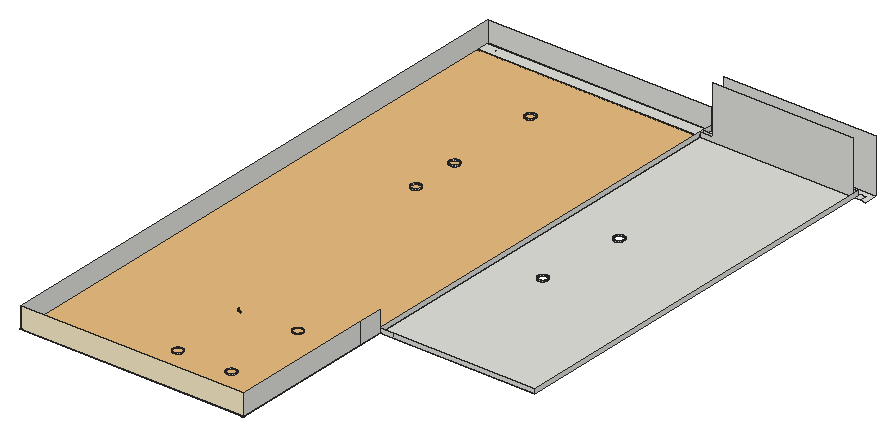
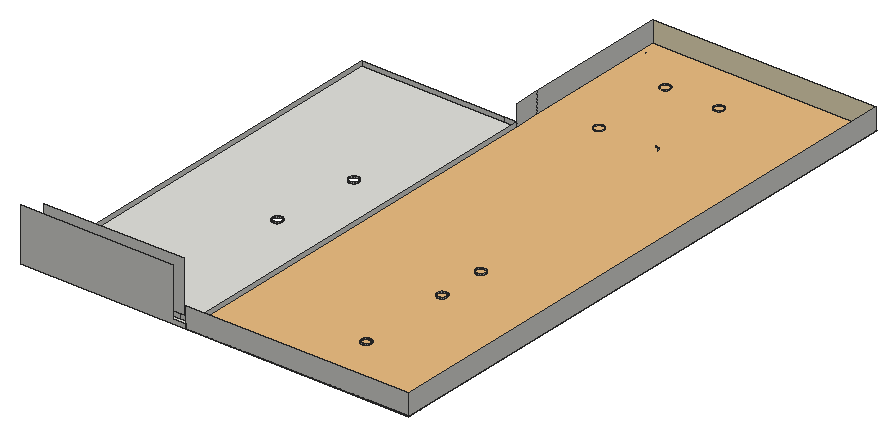
# SketchUp Ruby script. Lengths in inches.
U = 1.inch
M = Sketchup.active_model
def pt(a) = Geom::Point3d.new(a.map { |v| v * U })
def face(e, loops, mat)
  f = e.add_face(loops[0].map { |a| pt(a) })
  loops[1..].each { |l| e.add_face(l.map { |a| pt(a) }).erase! }
  f.material = f.back_material = mat if mat
  f
end
# faces: each face lists its corners as indices into pts; further lists are holes
def faces(e, pts, list, mat = nil) = list.each { |f| face(e, (f[0].is_a?(Array) ? f : [f]).map { |l| l.map { |i| pts[i] } }, mat) }
# xy, xz, yz: faces in a plane at the given z, y or x. An outline is a flat list of corners, or four numbers for a rectangle; further outlines are holes
def ring(l) = l.size == 4 ? [[l[0], l[1]], [l[2], l[1]], [l[2], l[3]], [l[0], l[3]]] : l.each_slice(2).to_a
def flat(e, list, mat, &to3) = list.each { |f| face(e, (f[0].is_a?(Array) ? f : [f]).map { |l| ring(l).map { |u, v| to3.(u, v) } }, mat) }
def xy(e, z, list, mat = nil) = flat(e, list, mat) { |x, y| [x, y, z] }
def xz(e, y, list, mat = nil) = flat(e, list, mat) { |x, z| [x, y, z] }
def yz(e, x, list, mat = nil) = flat(e, list, mat) { |y, z| [x, y, z] }
def lines(e, pts, list) = list.each { |a, b| e.add_line(pt(pts[a]), pt(pts[b])) }
# prism: a flat outline (further loops are holes) pulled along v
def prism(e, loops, v, mat = nil)
  f = face(e, loops, mat); d = Geom::Vector3d.new(v.map { |x| x * U })
  f.pushpull(f.normal.samedirection?(d) ? d.length : -d.length)
end
def box(e, o, s, mat = nil) = prism(e, [[o, [o[0] + s[0], o[1], o[2]], [o[0] + s[0], o[1] + s[1], o[2]], [o[0], o[1] + s[1], o[2]]]], [0, 0, s[2]], mat)
def at(x, y, z, deg = 0) = Geom::Transformation.translation(pt([x, y, z])) * Geom::Transformation.rotation(ORIGIN, Z_AXIS, deg.degrees)
def axes(o, x, y, z) = Geom::Transformation.new([*x, 0, *y, 0, *z, 0, *pt(o).to_a, 1])
def part(name) = M.definitions.add(name)
# library, detail: a bought-in or finely detailed component or shape, given as its bounding box
def library(name, o, s) = part(name).tap { |d| box(d.entities, o, s) }
def detail(e, o, s) = box(e.add_group.entities, o, s)
def put(e, d, t, mat = nil) = e.add_instance(d, t).tap { |i| i.material = mat if mat }
def group(e, t, mat = nil) = e.add_group.tap { |g| g.transformation = t; g.material = mat if mat }.entities
root = M.entities
M.materials.add("[Color D01]").color = [255, 242, 204]
M.materials.add("[Wood Veneer 01]").color = [120, 70, 37]
c1 = library("Mesh Light",[-0.5,-0.5,-0.1],[1,1,0.2])
xy(root,378,[[177.75,1087.125,177.75,1103.3125,657.75,1103.3125,657.75,1087.125,651,1087.125,651,1096.57,193.12,1096.57,193.12,1087.125],[193.12,1087.125,651,1096.57]])
xy(root,378,[[[183.75,402.08,183.75,631.27,189.75,631.27,189.75,593.57,206.9375,593.57,206.9375,683.82,416.0625,683.82,416.0625,593.57,446,593.57,446,402.08],[274.17,540.64,275.72,540.85,277.17,541.45,278.41,542.4,279.36,543.64,279.96,545.09,280.17,546.64,279.96,548.2,279.36,549.64,278.41,550.89,277.17,551.84,275.72,552.4375,274.17,552.64,272.61,552.4375,271.17,551.84,269.92,550.89,268.97,549.64,268.37,548.2,268.17,546.64,268.37,545.09,268.97,543.64,269.92,542.4,271.17,541.45,272.61,540.85],[388.79,540.64,390.34,540.85,391.79,541.45,393.03,542.4,393.99,543.64,394.59,545.09,394.79,546.64,394.59,548.2,393.99,549.64,393.03,550.89,391.79,551.84,390.34,552.4375,388.79,552.64,387.24,552.4375,385.79,551.84,384.55,550.89,383.59,549.64,382.99,548.2,382.79,546.64,382.99,545.09,383.59,543.64,384.55,542.4,385.79,541.45,387.24,540.85],[322.79,540.64,324.34,540.85,325.79,541.45,327.03,542.4,327.99,543.64,328.59,545.09,328.79,546.64,328.59,548.2,327.99,549.64,327.03,550.89,325.79,551.84,324.34,552.4375,322.79,552.64,321.24,552.4375,319.79,551.84,318.55,550.89,317.59,549.64,316.99,548.2,316.79,546.64,316.99,545.09,317.59,543.64,318.55,542.4,319.79,541.45,321.24,540.85],[223.8125,438.06,225.37,438.27,226.81,438.87,228.05,439.83,229,441.08,229.59,442.52,229.79,444.08,229.58,445.63,228.98,447.08,228.02,448.3125,226.77,449.26,225.32,449.86,223.77,450.06,222.22,449.84,220.77,449.24,219.53,448.28,218.58,447.04,217.99,445.59,217.79,444.03,218,442.48,218.61,441.04,219.5625,439.8,220.8125,438.85,222.26,438.25],[223.79,540.64,225.34,540.85,226.79,541.45,228.03,542.4,228.99,543.64,229.59,545.09,229.79,546.64,229.59,548.2,228.99,549.64,228.03,550.89,226.79,551.84,225.34,552.4375,223.79,552.64,222.24,552.4375,220.79,551.84,219.55,550.89,218.59,549.64,217.99,548.2,217.79,546.64,217.99,545.09,218.59,543.64,219.55,542.4,220.79,541.45,222.24,540.85],[274.1875,438.06,275.74,438.27,277.19,438.87,278.42,439.83,279.375,441.08,279.97,442.52,280.17,444.08,279.96,445.63,279.35,447.08,278.39,448.3125,277.15,449.26,275.7,449.86,274.14,450.06,272.59,449.84,271.15,449.24,269.91,448.28,268.96,447.04,268.36,445.59,268.17,444.03,268.375,442.48,268.98,441.04,269.9375,439.8,271.1875,438.85,272.63,438.25],[322.8125,438.06,324.37,438.27,325.81,438.87,327.05,439.83,328,441.08,328.59,442.52,328.79,444.08,328.58,445.63,327.98,447.08,327.02,448.3125,325.77,449.26,324.32,449.86,322.77,450.06,321.22,449.84,319.77,449.24,318.53,448.28,317.58,447.04,316.99,445.59,316.79,444.03,317,442.48,317.61,441.04,318.5625,439.8,319.8125,438.85,321.26,438.25],[388.8125,438.06,390.37,438.27,391.81,438.87,393.05,439.83,394,441.08,394.59,442.52,394.79,444.08,394.58,445.63,393.98,447.08,393.02,448.3125,391.77,449.26,390.32,449.86,388.77,450.06,387.22,449.84,385.77,449.24,384.53,448.28,383.58,447.04,382.99,445.59,382.79,444.03,383,442.48,383.61,441.04,384.5625,439.8,385.8125,438.85,387.26,438.25]]],"[Wood Veneer 01]")
xy(root,378.5,[[[452.87,593.61,644.41,1091.4],[509.16,768.54,510.71,768.75,512.16,769.35,513.4,770.3,514.35,771.54,514.95,772.99,515.16,774.54,514.95,776.1,514.35,777.54,513.4,778.79,512.16,779.74,510.71,780.34,509.16,780.54,507.6,780.34,506.16,779.74,504.91,778.79,503.96,777.54,503.36,776.1,503.16,774.54,503.36,772.99,503.96,771.54,504.91,770.3,506.16,769.35,507.6,768.75],[517.6,875.67,519.15,875.87,520.6,876.47,521.84,877.42,522.79,878.67,523.39,880.11,523.6,881.67,523.39,883.22,522.79,884.67,521.84,885.91,520.6,886.86,519.15,887.46,517.6,887.67,516.04,887.46,514.6,886.86,513.35,885.91,512.4,884.67,511.8,883.22,511.6,881.67,511.8,880.11,512.4,878.67,513.35,877.42,514.6,876.47,516.04,875.87]],[177.75,1087.125,452.87,1103.3125]])
xz(root,383.3125,[[177.75,378.5,452.87,404.125]],"[Color D01]")
xz(root,593.61,[[452.87,378.5,469.08,384],[469.08,378.5,644.41,384]])
xz(root,1087.125,[[177.75,378,641.5625,378,641.5625,444,469.06,444,469.06,384,452.87,384,452.87,378.5,177.75,378.5]])
xz(root,1091.4,[[452.87,378.5,469.08,384],[469.08,378.5,644.41,384]])
xz(root,1103.3125,[[177.75,378,177.75,378.5,452.87,378.5,452.87,384,469.06,384,469.06,444,657.75,444,657.75,378],[177.75,378.5,452.87,404.125]])
yz(root,177.75,[[383.3125,378.5,1103.3125,404.125]])
yz(root,452.87,[[383.3125,378.5,562.125,404.125],[562.125,378.5,593.61,404.125],[593.61,378.5,1087.125,384],[1087.125,378.5,1091.4,384],[1091.4,378.5,1103.3125,384]])
yz(root,644.41,[[593.61,378.5,1091.4,384]])
p = [[322.8125,438.06,378],[321.26,438.25,378],[321.26,438.25,379.1875],[322.8125,438.06,379.1875],[324.37,438.27,378],[324.37,438.27,379.1875],
  [388.8125,438.06,378],[387.26,438.25,378],[387.26,438.25,379.1875],[388.8125,438.06,379.1875],[390.37,438.27,378],[390.37,438.27,379.1875],
  [319.8125,438.85,378],[319.8125,438.85,379.1875],[325.81,438.87,378],[325.81,438.87,379.1875],[385.8125,438.85,378],[385.8125,438.85,379.1875],
  [391.81,438.87,378],[391.81,438.87,379.1875],[318.5625,439.8,378],[318.5625,439.8,379.1875],[384.5625,439.8,378],[384.5625,439.8,379.1875],
  [327.05,439.83,378],[327.05,439.83,379.1875],[393.05,439.83,378],[393.05,439.83,379.1875],[317.61,441.04,378],[317.61,441.04,379.1875],
  [328,441.08,378],[328,441.08,379.1875],[383.61,441.04,378],[383.61,441.04,379.1875],[394,441.08,378],[394,441.08,379.1875],
  [317,442.48,378],[317,442.48,379.1875],[383,442.48,378],[383,442.48,379.1875],[328.59,442.52,378],[328.59,442.52,379.1875],
  [394.59,442.52,378],[394.59,442.52,379.1875],[316.79,444.03,378],[316.79,444.03,379.1875],[328.79,444.08,378],[328.79,444.08,379.1875],
  [382.79,444.03,378],[382.79,444.03,379.1875],[394.79,444.08,378],[394.79,444.08,379.1875],[316.99,445.59,378],[316.99,445.59,379.1875],
  [382.99,445.59,378],[382.99,445.59,379.1875],[328.58,445.63,378],[328.58,445.63,379.1875],[394.58,445.63,378],[394.58,445.63,379.1875],
  [317.58,447.04,378],[317.58,447.04,379.1875],[327.98,447.08,378],[327.98,447.08,379.1875],[383.58,447.04,378],[383.58,447.04,379.1875],
  [393.98,447.08,378],[393.98,447.08,379.1875],[318.53,448.28,378],[318.53,448.28,379.1875],[384.53,448.28,378],[384.53,448.28,379.1875],
  [327.02,448.3125,378],[327.02,448.3125,379.1875],[393.02,448.3125,378],[393.02,448.3125,379.1875],[319.77,449.24,378],[319.77,449.24,379.1875],
  [325.77,449.26,378],[325.77,449.26,379.1875],[385.77,449.24,378],[385.77,449.24,379.1875],[391.77,449.26,378],[391.77,449.26,379.1875],
  [321.22,449.84,378],[321.22,449.84,379.1875],[387.22,449.84,378],[387.22,449.84,379.1875],[324.32,449.86,378],[324.32,449.86,379.1875],
  [390.32,449.86,378],[390.32,449.86,379.1875],[322.77,450.06,378],[322.77,450.06,379.1875],[388.77,450.06,378],[388.77,450.06,379.1875],
  [322.79,540.64,378],[321.24,540.85,378],[321.24,540.85,379.1875],[322.79,540.64,379.1875],[388.79,540.64,378],[387.24,540.85,378],
  [387.24,540.85,379.1875],[388.79,540.64,379.1875],[390.34,540.85,378],[390.34,540.85,379.1875],[319.79,541.45,378],[319.79,541.45,379.1875],
  [385.79,541.45,378],[385.79,541.45,379.1875],[391.79,541.45,378],[391.79,541.45,379.1875],[318.55,542.4,378],[318.55,542.4,379.1875],
  [384.55,542.4,378],[384.55,542.4,379.1875],[393.03,542.4,378],[393.03,542.4,379.1875],[317.59,543.64,378],[317.59,543.64,379.1875],
  [383.59,543.64,378],[383.59,543.64,379.1875],[393.99,543.64,378],[393.99,543.64,379.1875],[316.99,545.09,378],[316.99,545.09,379.1875],
  [382.99,545.09,378],[382.99,545.09,379.1875],[394.59,545.09,378],[394.59,545.09,379.1875],[382.79,546.64,378],[382.79,546.64,379.1875],
  [394.79,546.64,378],[394.79,546.64,379.1875],[382.99,548.2,378],[382.99,548.2,379.1875],[394.59,548.2,378],[394.59,548.2,379.1875],
  [383.59,549.64,378],[383.59,549.64,379.1875],[393.99,549.64,378],[393.99,549.64,379.1875],[384.55,550.89,378],[384.55,550.89,379.1875],
  [393.03,550.89,378],[393.03,550.89,379.1875],[385.79,551.84,378],[385.79,551.84,379.1875],[391.79,551.84,378],[391.79,551.84,379.1875],
  [387.24,552.4375,378],[387.24,552.4375,379.1875],[390.34,552.4375,378],[390.34,552.4375,379.1875],[388.79,552.64,378],[388.79,552.64,379.1875],
  [509.16,768.54,378.5],[507.6,768.75,378.5],[507.6,768.75,380.125],[509.16,768.54,380.125],[510.71,768.75,378.5],[510.71,768.75,380.125],
  [506.16,769.35,378.5],[506.16,769.35,380.125],[512.16,769.35,378.5],[512.16,769.35,380.125],[504.91,770.3,378.5],[504.91,770.3,380.125],
  [513.4,770.3,378.5],[513.4,770.3,380.125],[503.96,771.54,378.5],[503.96,771.54,380.125],[514.35,771.54,378.5],[514.35,771.54,380.125],
  [503.36,772.99,378.5],[503.36,772.99,380.125],[514.95,772.99,378.5],[514.95,772.99,380.125],[503.16,774.54,378.5],[503.16,774.54,380.125],
  [515.16,774.54,378.5],[515.16,774.54,380.125],[503.36,776.1,378.5],[503.36,776.1,380.125],[514.95,776.1,378.5],[514.95,776.1,380.125],
  [503.96,777.54,378.5],[503.96,777.54,380.125],[514.35,777.54,378.5],[514.35,777.54,380.125],[504.91,778.79,378.5],[504.91,778.79,380.125],
  [513.4,778.79,378.5],[513.4,778.79,380.125],[506.16,779.74,378.5],[506.16,779.74,380.125],[512.16,779.74,378.5],[512.16,779.74,380.125],
  [507.6,780.34,378.5],[507.6,780.34,380.125],[510.71,780.34,378.5],[510.71,780.34,380.125],[509.16,780.54,378.5],[509.16,780.54,380.125],
  [300.91,832.72,378.5],[299.36,832.92,378.5],[299.36,832.92,380.0625],[300.91,832.72,380.0625],[302.46,832.92,378.5],[302.46,832.92,380.0625],
  [297.91,833.52,378.5],[297.91,833.52,380.0625],[303.91,833.52,378.5],[303.91,833.52,380.0625],[296.67,834.47,378.5],[296.67,834.47,380.0625],
  [305.15,834.47,378.5],[305.15,834.47,380.0625],[295.71,835.72,378.5],[295.71,835.72,380.0625],[306.1,835.72,378.5],[306.1,835.72,380.0625],
  [295.11,837.16,378.5],[295.11,837.16,380.0625],[306.7,837.16,378.5],[306.7,837.16,380.0625],[294.91,838.72,378.5],[294.91,838.72,380.0625],
  [306.91,838.72,378.5],[306.91,838.72,380.0625],[295.11,840.27,378.5],[295.11,840.27,380.0625],[306.7,840.27,378.5],[306.7,840.27,380.0625],
  [295.71,841.72,378.5],[295.71,841.72,380.0625],[306.1,841.72,378.5],[306.1,841.72,380.0625],[296.67,842.96,378.5],[296.67,842.96,380.0625],
  [305.15,842.96,378.5],[305.15,842.96,380.0625],[297.91,843.91,378.5],[297.91,843.91,380.0625],[303.91,843.91,378.5],[303.91,843.91,380.0625],
  [299.36,844.51,378.5],[299.36,844.51,380.0625],[302.46,844.51,378.5],[302.46,844.51,380.0625],[300.91,844.72,378.5],[300.91,844.72,380.0625],
  [517.6,875.67,378.5],[516.04,875.87,378.5],[516.04,875.87,380.125],[517.6,875.67,380.125],[519.15,875.87,378.5],[519.15,875.87,380.125],
  [514.6,876.47,378.5],[514.6,876.47,380.125],[520.6,876.47,378.5],[520.6,876.47,380.125],[513.35,877.42,378.5],[513.35,877.42,380.125],
  [521.84,877.42,378.5],[521.84,877.42,380.125],[512.4,878.67,378.5],[512.4,878.67,380.125],[522.79,878.67,378.5],[522.79,878.67,380.125],
  [511.8,880.11,378.5],[511.8,880.11,380.125],[523.39,880.11,378.5],[523.39,880.11,380.125],[511.6,881.67,378.5],[511.6,881.67,380.125],
  [523.6,881.67,378.5],[523.6,881.67,380.125],[511.8,883.22,378.5],[511.8,883.22,380.125],[523.39,883.22,378.5],[523.39,883.22,380.125],
  [512.4,884.67,378.5],[512.4,884.67,380.125],[522.79,884.67,378.5],[522.79,884.67,380.125],[513.35,885.91,378.5],[513.35,885.91,380.125],
  [521.84,885.91,378.5],[521.84,885.91,380.125],[514.6,886.86,378.5],[514.6,886.86,380.125],[520.6,886.86,378.5],[520.6,886.86,380.125],
  [516.04,887.46,378.5],[516.04,887.46,380.125],[519.15,887.46,378.5],[519.15,887.46,380.125],[517.6,887.67,378.5],[517.6,887.67,380.125],
  [300.91,892.28,378.5],[299.36,892.48,378.5],[299.36,892.48,380.0625],[300.91,892.28,380.0625],[302.46,892.48,378.5],[302.46,892.48,380.0625],
  [297.91,893.08,378.5],[297.91,893.08,380.0625],[303.91,893.08,378.5],[303.91,893.08,380.0625],[296.67,894.04,378.5],[296.67,894.04,380.0625],
  [305.15,894.04,378.5],[305.15,894.04,380.0625],[295.71,895.28,378.5],[295.71,895.28,380.0625],[306.1,895.28,378.5],[306.1,895.28,380.0625],
  [295.11,896.73,378.5],[295.11,896.73,380.0625],[306.7,896.73,378.5],[306.7,896.73,380.0625],[294.91,898.28,378.5],[294.91,898.28,380.0625],
  [306.91,898.28,378.5],[306.91,898.28,380.0625],[295.11,899.83,378.5],[295.11,899.83,380.0625],[306.7,899.83,378.5],[306.7,899.83,380.0625],
  [295.71,901.28,378.5],[295.71,901.28,380.0625],[306.1,901.28,378.5],[306.1,901.28,380.0625],[296.67,902.52,378.5],[296.67,902.52,380.0625],
  [305.15,902.52,378.5],[305.15,902.52,380.0625],[297.91,903.48,378.5],[297.91,903.48,380.0625],[303.91,903.48,378.5],[303.91,903.48,380.0625],
  [299.36,904.07,378.5],[299.36,904.07,380.0625],[302.46,904.07,378.5],[302.46,904.07,380.0625],[300.91,904.28,378.5],[300.91,904.28,380.0625],
  [300.91,1009.53,378.5],[299.36,1009.73,378.5],[299.36,1009.73,380.0625],[300.91,1009.53,380.0625],[302.46,1009.73,378.5],[302.46,1009.73,380.0625],
  [297.91,1010.33,378.5],[297.91,1010.33,380.0625],[303.91,1010.33,378.5],[303.91,1010.33,380.0625],[296.67,1011.29,378.5],[296.67,1011.29,380.0625],
  [305.15,1011.29,378.5],[305.15,1011.29,380.0625],[295.71,1012.53,378.5],[295.71,1012.53,380.0625],[306.1,1012.53,378.5],[306.1,1012.53,380.0625],
  [295.11,1013.98,378.5],[295.11,1013.98,380.0625],[306.7,1013.98,378.5],[306.7,1013.98,380.0625],[294.91,1015.53,378.5],[294.91,1015.53,380.0625],
  [306.91,1015.53,378.5],[306.91,1015.53,380.0625],[295.11,1017.08,378.5],[295.11,1017.08,380.0625],[306.7,1017.08,378.5],[306.7,1017.08,380.0625],
  [295.71,1018.53,378.5],[295.71,1018.53,380.0625],[306.1,1018.53,378.5],[306.1,1018.53,380.0625],[296.67,1019.77,378.5],[296.67,1019.77,380.0625],
  [305.15,1019.77,378.5],[305.15,1019.77,380.0625],[297.91,1020.73,378.5],[297.91,1020.73,380.0625],[303.91,1020.73,378.5],[303.91,1020.73,380.0625],
  [299.36,1021.32,378.5],[299.36,1021.32,380.0625],[302.46,1021.32,378.5],[302.46,1021.32,380.0625],[300.91,1021.53,378.5],[300.91,1021.53,380.0625]]
faces(root,p,[[0,1,2,3],[4,0,3,5],[6,7,8,9],[10,6,9,11],[1,12,13,2],[14,4,5,15],[7,16,17,8],[18,10,11,19],
  [12,20,21,13],[16,22,23,17],[24,14,15,25],[26,18,19,27],[20,28,29,21],[30,24,25,31],[22,32,33,23],[34,26,27,35],
  [28,36,37,29],[32,38,39,33],[40,30,31,41],[42,34,35,43],[36,44,45,37],[46,40,41,47],[38,48,49,39],[50,42,43,51],
  [44,52,53,45],[48,54,55,49],[56,46,47,57],[58,50,51,59],[52,60,61,53],[62,56,57,63],[54,64,65,55],[66,58,59,67],
  [60,68,69,61],[64,70,71,65],[72,62,63,73],[74,66,67,75],[68,76,77,69],[78,72,73,79],[70,80,81,71],[82,74,75,83],
  [76,84,85,77],[80,86,87,81],[88,78,79,89],[90,82,83,91],[84,92,93,85],[86,94,95,87],[92,88,89,93],[94,90,91,95],
  [96,97,98,99],[100,101,102,103],[104,100,103,105],[97,106,107,98],[101,108,109,102],[110,104,105,111],[106,112,113,107],[108,114,115,109],
  [116,110,111,117],[112,118,119,113],[114,120,121,115],[122,116,117,123],[118,124,125,119],[120,126,127,121],[128,122,123,129],[126,130,131,127],
  [132,128,129,133],[130,134,135,131],[136,132,133,137],[134,138,139,135],[140,136,137,141],[138,142,143,139],[144,140,141,145],[142,146,147,143],
  [148,144,145,149],[146,150,151,147],[152,148,149,153],[150,154,155,151],[154,152,153,155],[156,157,158,159],[160,156,159,161],[157,162,163,158],
  [164,160,161,165],[162,166,167,163],[168,164,165,169],[166,170,171,167],[172,168,169,173],[170,174,175,171],[176,172,173,177],[174,178,179,175],
  [180,176,177,181],[178,182,183,179],[184,180,181,185],[182,186,187,183],[188,184,185,189],[186,190,191,187],[192,188,189,193],[190,194,195,191],
  [196,192,193,197],[194,198,199,195],[200,196,197,201],[198,202,203,199],[202,200,201,203],[204,205,206,207],[208,204,207,209],[205,210,211,206],
  [212,208,209,213],[210,214,215,211],[216,212,213,217],[214,218,219,215],[220,216,217,221],[218,222,223,219],[224,220,221,225],[222,226,227,223],
  [228,224,225,229],[226,230,231,227],[232,228,229,233],[230,234,235,231],[236,232,233,237],[234,238,239,235],[240,236,237,241],[238,242,243,239],
  [244,240,241,245],[242,246,247,243],[248,244,245,249],[246,250,251,247],[250,248,249,251],[252,253,254,255],[256,252,255,257],[253,258,259,254],
  [260,256,257,261],[258,262,263,259],[264,260,261,265],[262,266,267,263],[268,264,265,269],[266,270,271,267],[272,268,269,273],[270,274,275,271],
  [276,272,273,277],[274,278,279,275],[280,276,277,281],[278,282,283,279],[284,280,281,285],[282,286,287,283],[288,284,285,289],[286,290,291,287],
  [292,288,289,293],[290,294,295,291],[296,292,293,297],[294,298,299,295],[298,296,297,299],[300,301,302,303],[304,300,303,305],[301,306,307,302],
  [308,304,305,309],[306,310,311,307],[312,308,309,313],[310,314,315,311],[316,312,313,317],[314,318,319,315],[320,316,317,321],[318,322,323,319],
  [324,320,321,325],[322,326,327,323],[328,324,325,329],[326,330,331,327],[332,328,329,333],[330,334,335,331],[336,332,333,337],[334,338,339,335],
  [340,336,337,341],[338,342,343,339],[344,340,341,345],[342,346,347,343],[346,344,345,347],[348,349,350,351],[352,348,351,353],[349,354,355,350],
  [356,352,353,357],[354,358,359,355],[360,356,357,361],[358,362,363,359],[364,360,361,365],[362,366,367,363],[368,364,365,369],[366,370,371,367],
  [372,368,369,373],[370,374,375,371],[376,372,373,377],[374,378,379,375],[380,376,377,381],[378,382,383,379],[384,380,381,385],[382,386,387,383],
  [388,384,385,389],[386,390,391,387],[392,388,389,393],[390,394,395,391],[394,392,393,395]])
g1 = group(root,at(177.75,383.3125,378.5))
xy(g1,0,[[[0,0,275.12,703.8125],[123.16,626.22,124.71,626.42,126.16,627.02,127.4,627.97,128.35,629.22,128.95,630.66,129.16,632.22,128.95,633.77,128.35,635.22,127.4,636.46,126.16,637.41,124.71,638.01,123.16,638.22,121.6,638.01,120.16,637.41,118.92,636.46,117.96,635.22,117.36,633.77,117.16,632.22,117.36,630.66,117.96,629.22,118.92,627.97,120.16,627.02,121.6,626.42],[123.16,508.97,124.71,509.17,126.16,509.77,127.4,510.72,128.35,511.97,128.95,513.41,129.16,514.97,128.95,516.52,128.35,517.97,127.4,519.21,126.16,520.16,124.71,520.76,123.16,520.97,121.6,520.76,120.16,520.16,118.92,519.21,117.96,517.97,117.36,516.52,117.16,514.97,117.36,513.41,117.96,511.97,118.92,510.72,120.16,509.77,121.6,509.17],[123.16,449.4,124.71,449.61,126.16,450.21,127.4,451.16,128.35,452.4,128.95,453.85,129.16,455.4,128.95,456.96,128.35,458.4,127.4,459.65,126.16,460.6,124.71,461.2,123.16,461.4,121.6,461.2,120.16,460.6,118.92,459.65,117.96,458.4,117.36,456.96,117.16,455.4,117.36,453.85,117.96,452.4,118.92,451.16,120.16,450.21,121.6,449.61]]])
put(g1,c1,axes([137.56,351.91,0],[276.11866,0,0],[0,704.8125,0],[0,0,1]))
